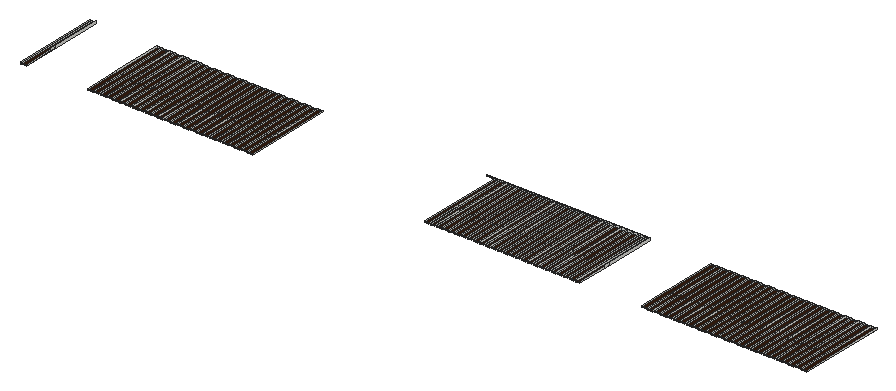
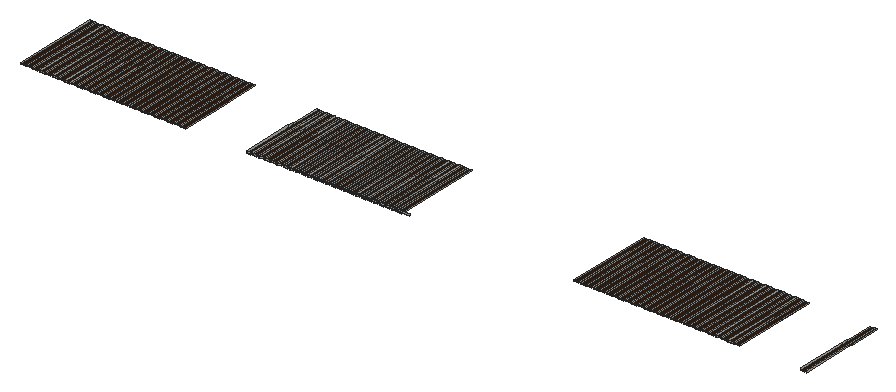
# SketchUp Ruby script. Lengths in inches.
U = 1.inch
M = Sketchup.active_model
def pt(a) = Geom::Point3d.new(a.map { |v| v * U })
def face(e, loops, mat)
  f = e.add_face(loops[0].map { |a| pt(a) })
  loops[1..].each { |l| e.add_face(l.map { |a| pt(a) }).erase! }
  f.material = f.back_material = mat if mat
  f
end
# faces: each face lists its corners as indices into pts; further lists are holes
def faces(e, pts, list, mat = nil) = list.each { |f| face(e, (f[0].is_a?(Array) ? f : [f]).map { |l| l.map { |i| pts[i] } }, mat) }
# xy, xz, yz: faces in a plane at the given z, y or x. An outline is a flat list of corners, or four numbers for a rectangle; further outlines are holes
def ring(l) = l.size == 4 ? [[l[0], l[1]], [l[2], l[1]], [l[2], l[3]], [l[0], l[3]]] : l.each_slice(2).to_a
def flat(e, list, mat, &to3) = list.each { |f| face(e, (f[0].is_a?(Array) ? f : [f]).map { |l| ring(l).map { |u, v| to3.(u, v) } }, mat) }
def xy(e, z, list, mat = nil) = flat(e, list, mat) { |x, y| [x, y, z] }
def xz(e, y, list, mat = nil) = flat(e, list, mat) { |x, z| [x, y, z] }
def yz(e, x, list, mat = nil) = flat(e, list, mat) { |y, z| [x, y, z] }
def lines(e, pts, list) = list.each { |a, b| e.add_line(pt(pts[a]), pt(pts[b])) }
# prism: a flat outline (further loops are holes) pulled along v
def prism(e, loops, v, mat = nil)
  f = face(e, loops, mat); d = Geom::Vector3d.new(v.map { |x| x * U })
  f.pushpull(f.normal.samedirection?(d) ? d.length : -d.length)
end
def box(e, o, s, mat = nil) = prism(e, [[o, [o[0] + s[0], o[1], o[2]], [o[0] + s[0], o[1] + s[1], o[2]], [o[0], o[1] + s[1], o[2]]]], [0, 0, s[2]], mat)
def at(x, y, z, deg = 0) = Geom::Transformation.translation(pt([x, y, z])) * Geom::Transformation.rotation(ORIGIN, Z_AXIS, deg.degrees)
def axes(o, x, y, z) = Geom::Transformation.new([*x, 0, *y, 0, *z, 0, *pt(o).to_a, 1])
def part(name) = M.definitions.add(name)
# library, detail: a bought-in or finely detailed component or shape, given as its bounding box
def library(name, o, s) = part(name).tap { |d| box(d.entities, o, s) }
def detail(e, o, s) = box(e.add_group.entities, o, s)
def put(e, d, t, mat = nil) = e.add_instance(d, t).tap { |i| i.material = mat if mat }
def group(e, t, mat = nil) = e.add_group.tap { |g| g.transformation = t; g.material = mat if mat }.entities
root = M.entities
M.materials.add("[Wood Veneer 01]").color = [51, 28, 15]
xy(root,503.875,[[1043.51,246.64,1049,361.27],[1721.07,246.64,1726.56,361.27],[1729.07,246.64,1734.56,361.27],[1737.07,246.64,1742.56,361.27],[1745.07,246.64,1750.56,361.27],
  [1753.07,246.64,1758.56,361.27],[1761.07,246.64,1766.56,361.27],[1769.07,246.64,1774.56,361.27],[1777.07,246.64,1782.56,361.27]],"[Wood Veneer 01]")
xy(root,504,[[1638.56,283.7,1638.56,288.72,1639.21,288.63,1639.81,288.38,1640.33,287.98,1640.73,287.46,1640.98,286.86,1641.07,286.21,1640.98,285.56,1640.73,284.95,1640.33,284.43,1639.81,284.03,1639.21,283.78]])
xy(root,504,[[1130.14,246.64,1136.84,361.27],[1138.64,246.64,1145.34,361.27],[1147.14,246.64,1153.84,361.27],[1155.64,246.64,1162.34,361.27],[1164.14,246.64,1170.84,361.27],
  [1172.64,246.64,1179.34,361.27],[1181.14,246.64,1187.84,361.27],[1189.64,246.64,1196.34,361.27],[1198.14,246.64,1204.84,361.27],[1206.64,246.64,1213.34,361.27],
  [1215.14,246.64,1221.84,361.27],[1223.64,246.64,1230.34,361.27],[1232.14,246.64,1238.84,361.27],[1240.64,246.64,1247.34,361.27],[1249.14,246.64,1255.84,361.27],
  [1257.64,246.64,1264.34,361.27],[1266.14,246.64,1272.84,361.27],[1274.64,246.64,1281.34,361.27],[1283.14,246.64,1289.84,361.27],[1291.64,246.64,1298.34,361.27],
  [1300.14,246.64,1306.84,361.27],[1308.64,246.64,1315.34,361.27],[1317.14,246.64,1323.84,361.27],[1325.64,246.64,1332.34,361.27],[1334.14,246.64,1340.84,361.27],
  [1342.64,246.64,1349.34,361.27],[1577.07,246.64,1582.56,361.27],[1585.07,246.64,1590.56,361.27],[1593.07,246.64,1598.56,361.27],[1601.07,246.64,1606.56,361.27],
  [1609.07,246.64,1614.56,361.27],[1617.07,246.64,1622.56,361.27],[1625.07,246.64,1630.56,361.27],[1633.07,246.64,1633.07,361.27,1638.56,361.27,1638.56,288.72,1637.91,288.63,1637.3,288.38,1636.78,287.98,1636.39,287.46,1636.14,286.86,1636.05,286.21,1636.14,285.56,1636.39,284.95,1636.78,284.43,1637.3,284.03,1637.91,283.78,1638.56,283.7,1638.56,246.64],[1641.07,246.64,1646.56,361.27],
  [1649.07,246.64,1654.56,361.27],[1657.07,246.64,1662.56,361.27],[1665.07,246.64,1670.56,361.27],[1673.07,246.64,1678.56,361.27],[1681.07,246.64,1686.56,361.27],
  [1689.07,246.64,1694.56,361.27],[1697.07,246.64,1702.56,361.27],[1705.07,246.64,1710.56,361.27],[1713.07,246.64,1718.56,361.27],[1863.7,246.64,1870.4,361.27],
  [1872.2,246.64,1878.9,361.27],[1880.7,246.64,1887.4,361.27],[1889.2,246.64,1895.9,361.27],[1897.7,246.64,1904.4,361.27],[1906.2,246.64,1912.9,361.27],
  [1914.7,246.64,1921.4,361.27],[1923.2,246.64,1929.9,361.27],[1931.7,246.64,1938.4,361.27],[1940.2,246.64,1946.9,361.27],[1948.7,246.64,1955.4,361.27],
  [1957.2,246.64,1963.9,361.27],[1965.7,246.64,1972.4,361.27],[1974.2,246.64,1980.9,361.27],[1982.7,246.64,1989.4,361.27],[1991.2,246.64,1997.9,361.27],
  [1999.7,246.64,2006.4,361.27],[2008.2,246.64,2014.9,361.27],[2016.7,246.64,2023.4,361.27],[2025.2,246.64,2031.9,361.27],[2033.7,246.64,2040.4,361.27],
  [2042.2,246.64,2048.9,361.27],[2050.7,246.64,2057.4,361.27],[2059.2,246.64,2065.9,361.27],[2067.7,246.64,2074.4,361.27],[2076.2,246.64,2082.9,361.27],
  [1638.56,283.7,1637.91,283.78,1637.3,284.03,1636.78,284.43,1636.39,284.95,1636.14,285.56,1636.05,286.21,1636.14,286.86,1636.39,287.46,1636.78,287.98,1637.3,288.38,1637.91,288.63,1638.56,288.72]],"[Wood Veneer 01]")
xz(root,246.64,[[1043.51,503.875,1049,503.875,1049,505.3125,1043.51,505.3],[1721.07,503.875,1726.56,505.1875],[1729.07,503.875,1734.56,503.875,1734.56,505.21,1729.07,505.19],[1737.07,503.875,1742.56,503.875,1742.56,505.22,1737.07,505.21],[1745.07,503.875,1750.56,503.875,1750.56,505.24,1745.07,505.23],
  [1753.07,503.875,1758.56,503.875,1758.56,505.26,1753.07,505.25],[1761.07,503.875,1766.56,503.875,1766.56,505.28,1761.07,505.26],[1769.07,503.875,1774.56,503.875,1774.56,505.29,1769.07,505.28],[1777.07,503.875,1782.56,503.875,1782.56,505.3125,1777.07,505.3],[1130.14,504,1136.84,505.3125],
  [1138.64,504,1145.34,505.3125],[1147.14,504,1153.84,505.3125],[1155.64,504,1162.34,505.3125],[1164.14,504,1170.84,505.3125],[1172.64,504,1179.34,505.3125],
  [1181.14,504,1187.84,505.3125],[1189.64,504,1196.34,505.3125],[1198.14,504,1204.84,505.3125],[1206.64,504,1213.34,505.3125],[1215.14,504,1221.84,505.3125],
  [1223.64,504,1230.34,505.3125],[1232.14,504,1238.84,505.3125],[1240.64,504,1247.34,505.3125],[1249.14,504,1255.84,505.3125],[1257.64,504,1264.34,505.3125],
  [1266.14,504,1272.84,505.3125],[1274.64,504,1281.34,505.3125],[1283.14,504,1289.84,505.3125],[1291.64,504,1298.34,505.3125],[1300.14,504,1306.84,505.3125],
  [1308.64,504,1315.34,505.3125],[1317.14,504,1323.84,505.3125],[1325.64,504,1332.34,505.3125],[1334.14,504,1340.84,505.3125],[1342.64,504,1349.34,505.3125],
  [1577.07,504,1582.56,505.3125],[1585.07,504,1590.56,505.3125],[1593.07,504,1598.56,505.3125],[1601.07,504,1606.56,505.3125],[1609.07,504,1614.56,505.3125],
  [1617.07,504,1622.56,505.3125],[1625.07,504,1630.56,505.3125],[1633.07,504,1638.56,505.3125],[1641.07,504,1646.56,505.3125],[1649.07,504,1654.56,505.3125],
  [1657.07,504,1662.56,505.3125],[1665.07,504,1670.56,505.3125],[1673.07,504,1678.56,505.3125],[1681.07,504,1686.56,505.3125],[1689.07,504,1694.56,505.3125],
  [1697.07,504,1702.56,505.3125],[1705.07,504,1710.56,505.3125],[1713.07,504,1718.56,505.3125],[1863.7,504,1870.4,505.3125],[1872.2,504,1878.9,505.3125],
  [1880.7,504,1887.4,505.3125],[1889.2,504,1895.9,505.3125],[1897.7,504,1904.4,505.3125],[1906.2,504,1912.9,505.3125],[1914.7,504,1921.4,505.3125],
  [1923.2,504,1929.9,505.3125],[1931.7,504,1938.4,505.3125],[1940.2,504,1946.9,505.3125],[1948.7,504,1955.4,505.3125],[1957.2,504,1963.9,505.3125],
  [1965.7,504,1972.4,505.3125],[1974.2,504,1980.9,505.3125],[1982.7,504,1989.4,505.3125],[1991.2,504,1997.9,505.3125],[1999.7,504,2006.4,505.3125],
  [2008.2,504,2014.9,505.3125],[2016.7,504,2023.4,505.3125],[2025.2,504,2031.9,505.3125],[2033.7,504,2040.4,505.3125],[2042.2,504,2048.9,505.3125],
  [2050.7,504,2057.4,505.3125],[2059.2,504,2065.9,505.3125],[2067.7,504,2074.4,505.3125],[2076.2,504,2082.9,505.3125]],"[Wood Veneer 01]")
xz(root,361.27,[[1729.07,503.875,1734.56,503.875,1734.56,505.3125,1737.07,505.3125,1737.07,503.875,1742.56,503.875,1742.56,505.3125,1745.07,505.3125,1745.07,503.875,1750.56,503.875,1750.56,505.3125,1753.07,505.3125,1753.07,503.875,1758.56,503.875,1758.56,505.3125,1761.07,505.3125,1761.07,503.875,1766.56,503.875,1766.56,505.3125,1769.07,505.3125,1769.07,503.875,1774.56,503.875,1774.56,505.3125,1777.07,505.3125,1777.07,503.875,1782.56,503.875,1782.56,506.8125,1567.3,506.8125,1567.3,505.3125,1721.07,505.3125,1721.07,505.1875,1726.56,505.1875,1726.56,505.3125,1729.07,505.3125],[1721.07,503.875,1726.56,505.1875],[1130.14,504,1136.84,505.3125],[1138.64,504,1145.34,505.3125],[1147.14,504,1153.84,505.3125],
  [1155.64,504,1162.34,505.3125],[1164.14,504,1170.84,505.3125],[1172.64,504,1179.34,505.3125],[1181.14,504,1187.84,505.3125],[1189.64,504,1196.34,505.3125],
  [1198.14,504,1204.84,505.3125],[1206.64,504,1213.34,505.3125],[1215.14,504,1221.84,505.3125],[1223.64,504,1230.34,505.3125],[1232.14,504,1238.84,505.3125],
  [1240.64,504,1247.34,505.3125],[1249.14,504,1255.84,505.3125],[1257.64,504,1264.34,505.3125],[1266.14,504,1272.84,505.3125],[1274.64,504,1281.34,505.3125],
  [1283.14,504,1289.84,505.3125],[1291.64,504,1298.34,505.3125],[1300.14,504,1306.84,505.3125],[1308.64,504,1315.34,505.3125],[1317.14,504,1323.84,505.3125],
  [1325.64,504,1332.34,505.3125],[1334.14,504,1340.84,505.3125],[1342.64,504,1348.32,505.3125],[1348.32,504,1349.34,505.3125],[1577.07,504,1582.56,505.3125],
  [1585.07,504,1590.56,505.3125],[1593.07,504,1598.56,505.3125],[1601.07,504,1606.56,505.3125],[1609.07,504,1614.56,505.3125],[1617.07,504,1622.56,505.3125],
  [1625.07,504,1630.56,505.3125],[1633.07,504,1638.56,505.3125],[1641.07,504,1646.56,505.3125],[1649.07,504,1654.56,505.3125],[1657.07,504,1662.56,505.3125],
  [1665.07,504,1670.56,505.3125],[1673.07,504,1678.56,505.3125],[1681.07,504,1686.56,505.3125],[1689.07,504,1694.56,505.3125],[1697.07,504,1702.56,505.3125],
  [1705.07,504,1710.56,505.3125],[1713.07,504,1718.56,505.3125],[1863.7,504,1870.4,505.3125],[1872.2,504,1878.9,505.3125],[1880.7,504,1887.4,505.3125],
  [1889.2,504,1895.9,505.3125],[1897.7,504,1904.4,505.3125],[1906.2,504,1912.9,505.3125],[1914.7,504,1921.4,505.3125],[1923.2,504,1929.9,505.3125],
  [1931.7,504,1938.4,505.3125],[1940.2,504,1946.9,505.3125],[1948.7,504,1955.4,505.3125],[1957.2,504,1963.9,505.3125],[1965.7,504,1972.4,505.3125],
  [1974.2,504,1980.9,505.3125],[1982.7,504,1989.4,505.3125],[1991.2,504,1997.9,505.3125],[1999.7,504,2006.4,505.3125],[2008.2,504,2014.9,505.3125],
  [2016.7,504,2023.4,505.3125],[2025.2,504,2031.9,505.3125],[2033.7,504,2040.4,505.3125],[2042.2,504,2048.9,505.3125],[2050.7,504,2057.4,505.3125],
  [2059.2,504,2065.9,505.3125],[2067.7,504,2074.4,505.3125],[2076.2,504,2081.89,505.3125],[2081.89,504,2082.9,505.3125]])
yz(root,1041,[[246.64,503.875,286.21,505.3125],[286.21,503.875,293.45,505.3125],[293.45,503.875,293.46,505.3125],[293.46,503.875,361.27,505.3125]])
yz(root,1043.51,[[246.64,503.875,361.27,505.3125]])
yz(root,1049,[[246.64,503.875,286.21,505.3125],[286.21,503.875,293.45,506.8125],[293.45,503.875,293.46,506.8125],[293.46,503.875,361.27,506.8125]])
yz(root,1130.14,[[246.64,504,286.21,505.3125],[286.21,504,293.45,505.3125],[293.45,504,361.27,505.3125]])
yz(root,1136.84,[[246.64,504,361.27,505.3125]])
yz(root,1138.64,[[246.64,504,286.21,505.3125],[286.21,504,293.45,505.3125],[293.45,504,361.27,505.3125]])
yz(root,1145.34,[[246.64,504,361.27,505.3125]])
yz(root,1147.14,[[246.64,504,286.21,505.3125],[286.21,504,293.45,505.3125],[293.45,504,361.27,505.3125]])
yz(root,1153.84,[[246.64,504,361.27,505.3125]])
yz(root,1155.64,[[246.64,504,286.21,505.3125],[286.21,504,293.45,505.3125],[293.45,504,361.27,505.3125]])
yz(root,1162.34,[[246.64,504,361.27,505.3125]])
yz(root,1164.14,[[246.64,504,286.21,505.3125],[286.21,504,293.45,505.3125],[293.45,504,361.27,505.3125]])
yz(root,1170.84,[[246.64,504,361.27,505.3125]])
yz(root,1172.64,[[246.64,504,286.21,505.3125],[286.21,504,293.45,505.3125],[293.45,504,361.27,505.3125]])
yz(root,1179.34,[[246.64,504,361.27,505.3125]])
yz(root,1181.14,[[246.64,504,286.21,505.3125],[286.21,504,293.45,505.3125],[293.45,504,361.27,505.3125]])
yz(root,1187.84,[[246.64,504,361.27,505.3125]])
yz(root,1189.64,[[246.64,504,286.21,505.3125],[286.21,504,293.45,505.3125],[293.45,504,361.27,505.3125]])
yz(root,1196.34,[[246.64,504,361.27,505.3125]])
yz(root,1198.14,[[246.64,504,286.21,505.3125],[286.21,504,293.45,505.3125],[293.45,504,361.27,505.3125]])
yz(root,1204.84,[[246.64,504,361.27,505.3125]])
yz(root,1206.64,[[246.64,504,286.21,505.3125],[286.21,504,293.45,505.3125],[293.45,504,361.27,505.3125]])
yz(root,1213.34,[[246.64,504,361.27,505.3125]])
yz(root,1215.14,[[246.64,504,286.21,505.3125],[286.21,504,293.45,505.3125],[293.45,504,361.27,505.3125]])
yz(root,1221.84,[[246.64,504,361.27,505.3125]])
yz(root,1223.64,[[246.64,504,286.21,505.3125],[286.21,504,293.45,505.3125],[293.45,504,361.27,505.3125]])
yz(root,1230.34,[[246.64,504,361.27,505.3125]])
yz(root,1232.14,[[246.64,504,286.21,505.3125],[286.21,504,293.45,505.3125],[293.45,504,361.27,505.3125]])
yz(root,1238.84,[[246.64,504,361.27,505.3125]])
yz(root,1240.64,[[246.64,504,286.21,505.3125],[286.21,504,293.45,505.3125],[293.45,504,361.27,505.3125]])
yz(root,1247.34,[[246.64,504,361.27,505.3125]])
yz(root,1249.14,[[246.64,504,286.21,505.3125],[286.21,504,293.45,505.3125],[293.45,504,361.27,505.3125]])
yz(root,1255.84,[[246.64,504,361.27,505.3125]])
yz(root,1257.64,[[246.64,504,286.21,505.3125],[286.21,504,293.45,505.3125],[293.45,504,361.27,505.3125]])
yz(root,1264.34,[[246.64,504,361.27,505.3125]])
yz(root,1266.14,[[246.64,504,286.21,505.3125],[286.21,504,293.45,505.3125],[293.45,504,361.27,505.3125]])
yz(root,1272.84,[[246.64,504,361.27,505.3125]])
yz(root,1274.64,[[246.64,504,286.21,505.3125],[286.21,504,293.45,505.3125],[293.45,504,361.27,505.3125]])
yz(root,1281.34,[[246.64,504,361.27,505.3125]])
yz(root,1283.14,[[246.64,504,286.21,505.3125],[286.21,504,293.45,505.3125],[293.45,504,361.27,505.3125]])
yz(root,1289.84,[[246.64,504,361.27,505.3125]])
yz(root,1291.64,[[246.64,504,286.21,505.3125],[286.21,504,293.45,505.3125],[293.45,504,361.27,505.3125]])
yz(root,1298.34,[[246.64,504,361.27,505.3125]])
yz(root,1300.14,[[246.64,504,286.21,505.3125],[286.21,504,293.45,505.3125],[293.45,504,361.27,505.3125]])
yz(root,1306.84,[[246.64,504,361.27,505.3125]])
yz(root,1308.64,[[246.64,504,286.21,505.3125],[286.21,504,293.45,505.3125],[293.45,504,361.27,505.3125]])
yz(root,1315.34,[[246.64,504,361.27,505.3125]])
yz(root,1317.14,[[246.64,504,286.21,505.3125],[286.21,504,293.45,505.3125],[293.45,504,361.27,505.3125]])
yz(root,1323.84,[[246.64,504,361.27,505.3125]])
yz(root,1325.64,[[246.64,504,286.21,505.3125],[286.21,504,293.45,505.3125],[293.45,504,361.27,505.3125]])
yz(root,1332.34,[[246.64,504,361.27,505.3125]])
yz(root,1334.14,[[246.64,504,286.21,505.3125],[286.21,504,293.45,505.3125],[293.45,504,361.27,505.3125]])
yz(root,1340.84,[[246.64,504,361.27,505.3125]])
yz(root,1342.64,[[246.64,504,286.21,505.3125],[286.21,504,293.45,505.3125],[293.45,504,361.27,505.3125]])
yz(root,1349.34,[[246.64,504,361.27,505.3125]])
yz(root,1577.07,[[246.64,504,361.27,505.3125]])
yz(root,1582.56,[[246.64,504,286.21,505.3125],[286.21,504,293.45,505.3125],[293.45,504,293.46,505.3125],[293.46,504,361.27,505.3125]])
yz(root,1585.07,[[246.64,504,361.27,505.3125]])
yz(root,1590.56,[[246.64,504,286.21,505.3125],[286.21,504,293.45,505.3125],[293.45,504,293.46,505.3125],[293.46,504,361.27,505.3125]])
yz(root,1593.07,[[246.64,504,361.27,505.3125]])
yz(root,1598.56,[[246.64,504,286.21,505.3125],[286.21,504,293.45,505.3125],[293.45,504,293.46,505.3125],[293.46,504,361.27,505.3125]])
yz(root,1601.07,[[246.64,504,361.27,505.3125]])
yz(root,1606.56,[[246.64,504,286.21,505.3125],[286.21,504,293.45,505.3125],[293.45,504,293.46,505.3125],[293.46,504,361.27,505.3125]])
yz(root,1609.07,[[246.64,504,361.27,505.3125]])
yz(root,1614.56,[[246.64,504,286.21,505.3125],[286.21,504,293.45,505.3125],[293.45,504,293.46,505.3125],[293.46,504,361.27,505.3125]])
yz(root,1617.07,[[246.64,504,361.27,505.3125]])
yz(root,1622.56,[[246.64,504,286.21,505.3125],[286.21,504,293.45,505.3125],[293.45,504,293.46,505.3125],[293.46,504,361.27,505.3125]])
yz(root,1625.07,[[246.64,504,361.27,505.3125]])
yz(root,1630.56,[[246.64,504,286.21,505.3125],[286.21,504,293.45,505.3125],[293.45,504,293.46,505.3125],[293.46,504,361.27,505.3125]])
yz(root,1633.07,[[246.64,504,361.27,505.3125]])
yz(root,1638.56,[[246.64,504,286.21,505.3125],[286.21,504,293.45,505.3125],[293.45,504,293.46,505.3125],[293.46,504,361.27,505.3125]])
yz(root,1641.07,[[246.64,504,361.27,505.3125]])
yz(root,1646.56,[[246.64,504,286.21,505.3125],[286.21,504,293.45,505.3125],[293.45,504,293.46,505.3125],[293.46,504,361.27,505.3125]])
yz(root,1649.07,[[246.64,504,361.27,505.3125]])
yz(root,1654.56,[[246.64,504,286.21,505.3125],[286.21,504,293.45,505.3125],[293.45,504,293.46,505.3125],[293.46,504,361.27,505.3125]])
yz(root,1657.07,[[246.64,504,361.27,505.3125]])
yz(root,1662.56,[[246.64,504,286.21,505.3125],[286.21,504,293.45,505.3125],[293.45,504,293.46,505.3125],[293.46,504,361.27,505.3125]])
yz(root,1665.07,[[246.64,504,361.27,505.3125]])
yz(root,1670.56,[[246.64,504,286.21,505.3125],[286.21,504,293.45,505.3125],[293.45,504,293.46,505.3125],[293.46,504,361.27,505.3125]])
yz(root,1673.07,[[246.64,504,361.27,505.3125]])
yz(root,1678.56,[[246.64,504,286.21,505.3125],[286.21,504,293.45,505.3125],[293.45,504,293.46,505.3125],[293.46,504,361.27,505.3125]])
yz(root,1681.07,[[246.64,504,361.27,505.3125]])
yz(root,1686.56,[[246.64,504,286.21,505.3125],[286.21,504,293.45,505.3125],[293.45,504,293.46,505.3125],[293.46,504,361.27,505.3125]])
yz(root,1689.07,[[246.64,504,361.27,505.3125]])
yz(root,1694.56,[[246.64,504,286.21,505.3125],[286.21,504,293.45,505.3125],[293.45,504,293.46,505.3125],[293.46,504,361.27,505.3125]])
yz(root,1697.07,[[246.64,504,361.27,505.3125]])
yz(root,1702.56,[[246.64,504,286.21,505.3125],[286.21,504,293.45,505.3125],[293.45,504,293.46,505.3125],[293.46,504,361.27,505.3125]])
yz(root,1705.07,[[246.64,504,361.27,505.3125]])
yz(root,1710.56,[[246.64,504,286.21,505.3125],[286.21,504,293.45,505.3125],[293.45,504,293.46,505.3125],[293.46,504,361.27,505.3125]])
yz(root,1713.07,[[246.64,504,361.27,505.3125]])
yz(root,1718.56,[[246.64,504,286.21,505.3125],[286.21,504,293.45,505.3125],[293.45,504,293.46,505.3125],[293.46,504,361.27,505.3125]])
yz(root,1721.07,[[246.64,503.875,361.27,505.1875]])
yz(root,1726.56,[[246.64,503.875,286.21,505.1875],[286.21,503.875,293.45,505.1875],[293.45,503.875,293.46,505.1875],[293.46,503.875,361.27,505.1875]])
yz(root,1729.07,[[246.64,503.875,361.27,505.3125]])
yz(root,1734.56,[[246.64,503.875,286.21,505.3125],[286.21,503.875,293.45,505.3125],[293.45,503.875,293.46,505.3125],[293.46,503.875,361.27,505.3125]])
yz(root,1737.07,[[246.64,503.875,361.27,505.3125]])
yz(root,1742.56,[[246.64,503.875,286.21,505.3125],[286.21,503.875,293.45,505.3125],[293.45,503.875,293.46,505.3125],[293.46,503.875,361.27,505.3125]])
yz(root,1745.07,[[246.64,503.875,361.27,505.3125]])
yz(root,1750.56,[[246.64,503.875,286.21,505.3125],[286.21,503.875,293.45,505.3125],[293.45,503.875,293.46,505.3125],[293.46,503.875,361.27,505.3125]])
yz(root,1753.07,[[246.64,503.875,361.27,505.3125]])
yz(root,1758.56,[[246.64,503.875,286.21,505.3125],[286.21,503.875,293.45,505.3125],[293.45,503.875,293.46,505.3125],[293.46,503.875,361.27,505.3125]])
yz(root,1761.07,[[246.64,503.875,361.27,505.3125]])
yz(root,1766.56,[[246.64,503.875,286.21,505.3125],[286.21,503.875,293.45,505.3125],[293.45,503.875,293.46,505.3125],[293.46,503.875,361.27,505.3125]])
yz(root,1769.07,[[246.64,503.875,361.27,505.3125]])
yz(root,1774.56,[[246.64,503.875,286.21,505.3125],[286.21,503.875,293.45,505.3125],[293.45,503.875,293.46,505.3125],[293.46,503.875,361.27,505.3125]])
yz(root,1777.07,[[246.64,503.875,361.27,505.3125]])
yz(root,1782.56,[[246.64,503.875,286.21,505.3125],[286.21,503.875,293.45,506.8125],[293.45,503.875,293.46,506.8125],[293.46,503.875,361.27,506.8125]])
yz(root,1863.7,[[246.64,504,286.21,505.3125],[286.21,504,293.45,505.3125],[293.45,504,361.27,505.3125]])
yz(root,1870.4,[[246.64,504,361.27,505.3125]])
yz(root,1872.2,[[246.64,504,286.21,505.3125],[286.21,504,293.45,505.3125],[293.45,504,361.27,505.3125]])
yz(root,1878.9,[[246.64,504,361.27,505.3125]])
yz(root,1880.7,[[246.64,504,286.21,505.3125],[286.21,504,293.45,505.3125],[293.45,504,361.27,505.3125]])
yz(root,1887.4,[[246.64,504,361.27,505.3125]])
yz(root,1889.2,[[246.64,504,286.21,505.3125],[286.21,504,293.45,505.3125],[293.45,504,361.27,505.3125]])
yz(root,1895.9,[[246.64,504,361.27,505.3125]])
yz(root,1897.7,[[246.64,504,286.21,505.3125],[286.21,504,293.45,505.3125],[293.45,504,361.27,505.3125]])
yz(root,1904.4,[[246.64,504,361.27,505.3125]])
yz(root,1906.2,[[246.64,504,286.21,505.3125],[286.21,504,293.45,505.3125],[293.45,504,361.27,505.3125]])
yz(root,1912.9,[[246.64,504,361.27,505.3125]])
yz(root,1914.7,[[246.64,504,286.21,505.3125],[286.21,504,293.45,505.3125],[293.45,504,361.27,505.3125]])
yz(root,1921.4,[[246.64,504,361.27,505.3125]])
yz(root,1923.2,[[246.64,504,286.21,505.3125],[286.21,504,293.45,505.3125],[293.45,504,361.27,505.3125]])
yz(root,1929.9,[[246.64,504,361.27,505.3125]])
yz(root,1931.7,[[246.64,504,286.21,505.3125],[286.21,504,293.45,505.3125],[293.45,504,361.27,505.3125]])
yz(root,1938.4,[[246.64,504,361.27,505.3125]])
yz(root,1940.2,[[246.64,504,286.21,505.3125],[286.21,504,293.45,505.3125],[293.45,504,361.27,505.3125]])
yz(root,1946.9,[[246.64,504,361.27,505.3125]])
yz(root,1948.7,[[246.64,504,286.21,505.3125],[286.21,504,293.45,505.3125],[293.45,504,361.27,505.3125]])
yz(root,1955.4,[[246.64,504,361.27,505.3125]])
yz(root,1957.2,[[246.64,504,286.21,505.3125],[286.21,504,293.45,505.3125],[293.45,504,361.27,505.3125]])
yz(root,1963.9,[[246.64,504,361.27,505.3125]])
yz(root,1965.7,[[246.64,504,286.21,505.3125],[286.21,504,293.45,505.3125],[293.45,504,361.27,505.3125]])
yz(root,1972.4,[[246.64,504,361.27,505.3125]])
yz(root,1974.2,[[246.64,504,286.21,505.3125],[286.21,504,293.45,505.3125],[293.45,504,361.27,505.3125]])
yz(root,1980.9,[[246.64,504,361.27,505.3125]])
yz(root,1982.7,[[246.64,504,286.21,505.3125],[286.21,504,293.45,505.3125],[293.45,504,361.27,505.3125]])
yz(root,1989.4,[[246.64,504,361.27,505.3125]])
yz(root,1991.2,[[246.64,504,286.21,505.3125],[286.21,504,293.45,505.3125],[293.45,504,361.27,505.3125]])
yz(root,1997.9,[[246.64,504,361.27,505.3125]])
yz(root,1999.7,[[246.64,504,286.21,505.3125],[286.21,504,293.45,505.3125],[293.45,504,361.27,505.3125]])
yz(root,2006.4,[[246.64,504,361.27,505.3125]])
yz(root,2008.2,[[246.64,504,286.21,505.3125],[286.21,504,293.45,505.3125],[293.45,504,361.27,505.3125]])
yz(root,2014.9,[[246.64,504,361.27,505.3125]])
yz(root,2016.7,[[246.64,504,286.21,505.3125],[286.21,504,293.45,505.3125],[293.45,504,361.27,505.3125]])
yz(root,2023.4,[[246.64,504,361.27,505.3125]])
yz(root,2025.2,[[246.64,504,286.21,505.3125],[286.21,504,293.45,505.3125],[293.45,504,361.27,505.3125]])
yz(root,2031.9,[[246.64,504,361.27,505.3125]])
yz(root,2033.7,[[246.64,504,286.21,505.3125],[286.21,504,293.45,505.3125],[293.45,504,361.27,505.3125]])
yz(root,2040.4,[[246.64,504,361.27,505.3125]])
yz(root,2042.2,[[246.64,504,286.21,505.3125],[286.21,504,293.45,505.3125],[293.45,504,361.27,505.3125]])
yz(root,2048.9,[[246.64,504,361.27,505.3125]])
yz(root,2050.7,[[246.64,504,286.21,505.3125],[286.21,504,293.45,505.3125],[293.45,504,361.27,505.3125]])
yz(root,2057.4,[[246.64,504,361.27,505.3125]])
yz(root,2059.2,[[246.64,504,286.21,505.3125],[286.21,504,293.45,505.3125],[293.45,504,361.27,505.3125]])
yz(root,2065.9,[[246.64,504,361.27,505.3125]])
yz(root,2067.7,[[246.64,504,286.21,505.3125],[286.21,504,293.45,505.3125],[293.45,504,361.27,505.3125]])
yz(root,2074.4,[[246.64,504,361.27,505.3125]])
yz(root,2076.2,[[246.64,504,286.21,505.3125],[286.21,504,293.45,505.3125],[293.45,504,361.27,505.3125]])
yz(root,2082.9,[[246.64,504,361.27,505.3125]])
